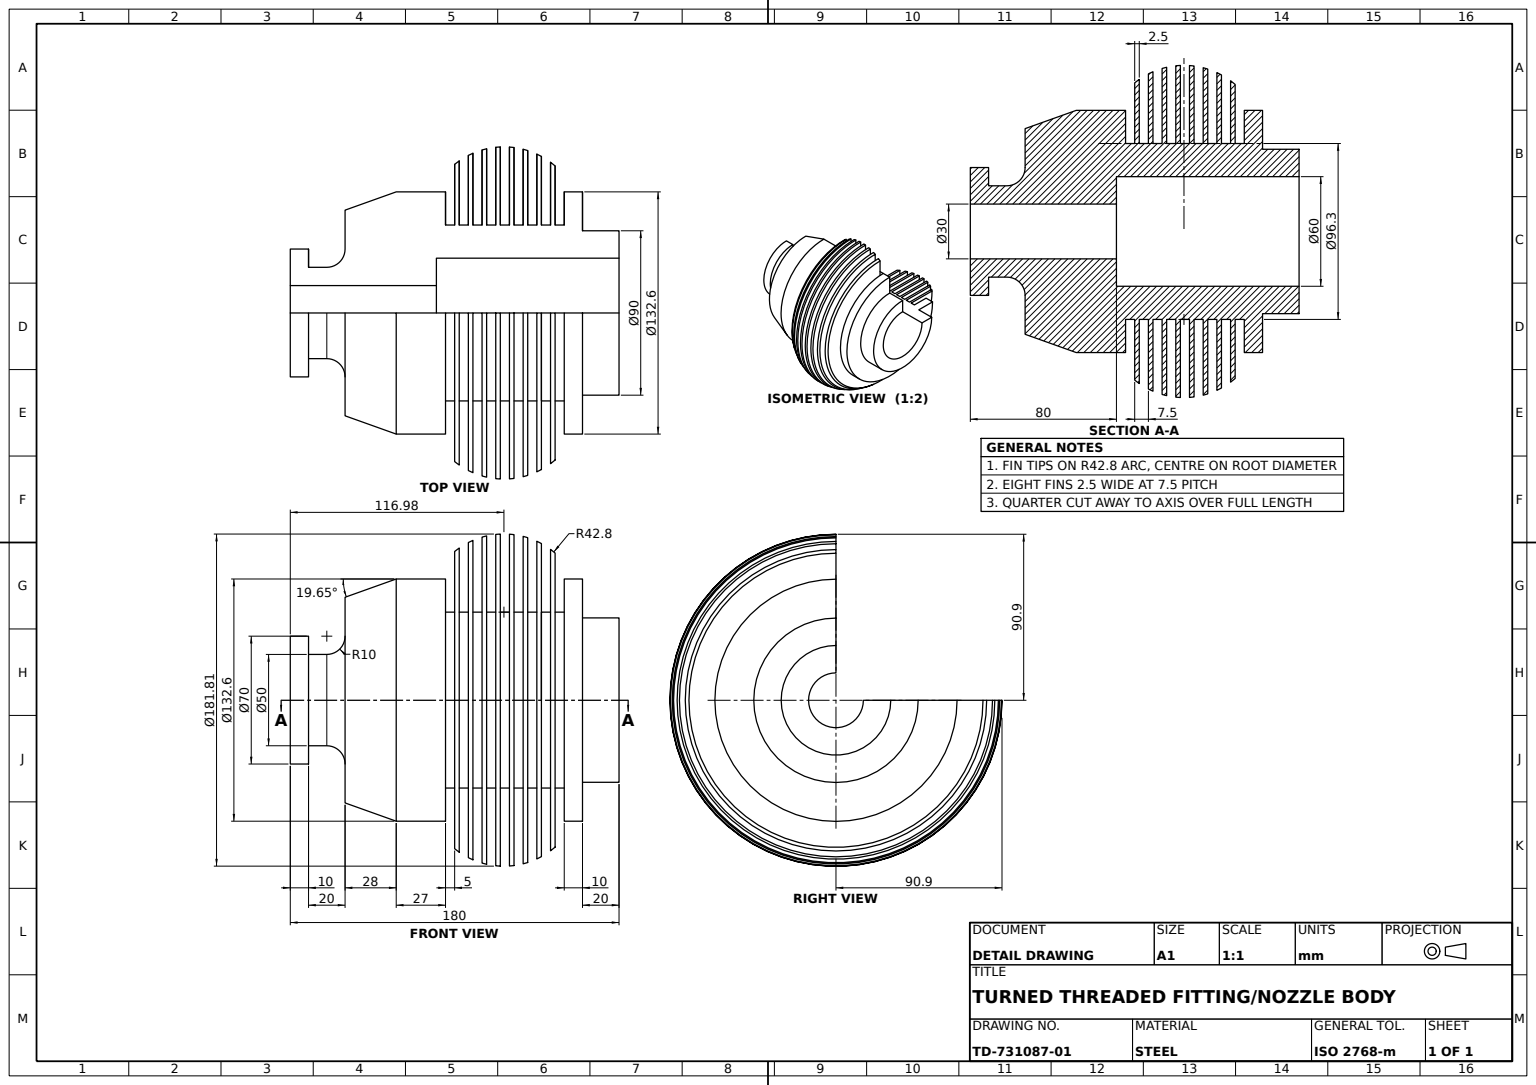
solid
v1 (31.156388,0,59.625514)
v2 (21.156388,0,59.625514)
e1 v1 v2 LINE
v3 (31.156388,66.3,-6.674486)
e2 v1 v3 CIRCLE(AX(P(31.156388,0,-6.674486),D(-1,0,0),D(0,0,1)),66.3)
v4 (21.156388,66.3,-6.674486)
e3 v3 v4 LINE
e4 v2 v4 CIRCLE(AX(P(21.156388,0,-6.674486),D(-1,0,0),D(0,0,1)),66.3)
face CYL(AX(P(-149.60578,0,-6.674486),D(-1,0,0),D(0,0,1)),66.3) [-e1 e2 e3 -e4]
v5 (-31.343612,0,41.475514)
v6 (-31.343612,48.15,-6.674486)
e5 v5 v6 CIRCLE(AX(P(-31.343612,0,-6.674486),D(-1,0,0),D(0,0,1)),48.15)
v7 (-36.343612,48.15,-6.674486)
e6 v7 v6 LINE
v8 (-36.343612,0,41.475514)
e7 v8 v7 CIRCLE(AX(P(-36.343612,0,-6.674486),D(-1,0,0),D(0,0,1)),48.15)
e8 v5 v8 LINE
face CYL(AX(P(-149.60578,0,-6.674486),D(-1,0,0),D(0,0,1)),48.15) [e5 -e6 -e7 -e8]
v9 (-13.843612,0,-54.824486)
v10 (-13.843612,0,41.475514)
e9 v9 v10 CIRCLE(AX(P(-13.843612,0,-6.674486),D(-1,0,0),D(0,0,1)),48.15)
v11 (-8.843612,0,-54.824486)
e10 v9 v11 LINE
v12 (-8.843612,0,41.475514)
e11 v11 v12 CIRCLE(AX(P(-8.843612,0,-6.674486),D(-1,0,0),D(0,0,1)),48.15)
e12 v12 v10 LINE
face CYL(AX(P(-149.60578,0,-6.674486),D(-1,0,0),D(0,0,1)),48.15) [-e9 e10 e11 e12]
v13 (-108.843612,0,18.325514)
v14 (-108.843612,25,-6.674486)
e13 v13 v14 CIRCLE(AX(P(-108.843612,0,-6.674486),D(-1,0,0),D(0,0,1)),25)
v15 (-98.843612,0,28.325514)
e14 v13 v15 CIRCLE(AX(P(-108.843612,0,28.325514),D(0,-1,0),D(0,0,-1)),10)
v16 (-98.843612,35,-6.674486)
e15 v15 v16 CIRCLE(AX(P(-98.843612,0,-6.674486),D(-1,0,0),D(0,0,1)),35)
e16 v16 v14 CIRCLE(AX(P(-108.843612,35,-6.674486),D(0,0,-1),D(1,0,0)),10)
face TORUS(AX(P(-108.843612,0,-6.674486),D(-1,0,0),D(0,0,1)),35,10) rev [-e13 e14 e15 e16]
v17 (6.156388,0,-54.824486)
v18 (6.156388,0,41.475514)
e17 v17 v18 CIRCLE(AX(P(6.156388,0,-6.674486),D(-1,0,0),D(0,0,1)),48.15)
v19 (1.156388,0,41.475514)
e18 v18 v19 LINE
v20 (1.156388,0,-54.824486)
e19 v20 v19 CIRCLE(AX(P(1.156388,0,-6.674486),D(-1,0,0),D(0,0,1)),48.15)
e20 v20 v17 LINE
face CYL(AX(P(-149.60578,0,-6.674486),D(-1,0,0),D(0,0,1)),48.15) [e17 e18 -e19 e20]
v21 (-128.843612,0,8.325514)
v22 (-128.843612,15,-6.674486)
e21 v21 v22 CIRCLE(AX(P(-128.843612,0,-6.674486),D(-1,0,0),D(0,0,1)),15)
v23 (-48.843612,15,-6.674486)
e22 v23 v22 LINE
v24 (-48.843612,0,8.325514)
e23 v24 v23 CIRCLE(AX(P(-48.843612,0,-6.674486),D(-1,0,0),D(0,0,1)),15)
e24 v24 v21 LINE
face CYL(AX(P(-149.60578,0,-6.674486),D(-1,0,0),D(0,0,1)),15) rev [e21 -e22 -e23 e24]
v25 (1.156388,0,-95.595676)
v26 (1.156388,0,82.246704)
e25 v25 v26 CIRCLE(AX(P(1.156388,0,-6.674486),D(-1,0,0),D(0,0,1)),88.92119)
e26 v25 v20 LINE
v27 (1.156388,48.15,-6.674486)
e27 v19 v27 CIRCLE(AX(P(1.156388,0,-6.674486),D(-1,0,0),D(0,0,1)),48.15)
v28 (1.156388,88.92119,-6.674486)
e28 v28 v27 LINE
e29 v26 v28 CIRCLE(AX(P(1.156388,0,-6.674486),D(-1,0,0),D(0,0,1)),88.92119)
face PLANE(AX(P(1.156388,0,0),D(1,0,0),D(0,0,-1))) [-e25 e26 e19 e27 -e28 -e29]
v29 (8.656388,0,79.035105)
v30 (8.656388,85.709591,-6.674486)
e30 v29 v30 CIRCLE(AX(P(8.656388,0,-6.674486),D(-1,0,0),D(0,0,1)),85.709591)
v31 (6.156388,86.97111,-6.674486)
e31 v30 v31 CIRCLE(AX(P(-11.86475,48.15,-6.674486),D(0,0,1),D(1,0,0)),42.8)
v32 (6.156388,0,80.296624)
e32 v32 v31 CIRCLE(AX(P(6.156388,0,-6.674486),D(-1,0,0),D(0,0,1)),86.97111)
e33 v29 v32 CIRCLE(AX(P(-11.86475,0,41.475514),D(0,-1,0),D(0,0,-1)),42.8)
face TORUS(AX(P(-11.86475,0,-6.674486),D(-1,0,0),D(0,0,1)),48.15,42.8) [e30 e31 -e32 -e33]
v33 (-6.343612,0,-54.824486)
v34 (-1.343612,0,-54.824486)
e34 v33 v34 LINE
v35 (-1.343612,0,41.475514)
e35 v34 v35 CIRCLE(AX(P(-1.343612,0,-6.674486),D(-1,0,0),D(0,0,1)),48.15)
v36 (-6.343612,0,41.475514)
e36 v35 v36 LINE
e37 v33 v36 CIRCLE(AX(P(-6.343612,0,-6.674486),D(-1,0,0),D(0,0,1)),48.15)
face CYL(AX(P(-149.60578,0,-6.674486),D(-1,0,0),D(0,0,1)),48.15) [e34 e35 e36 -e37]
v37 (-108.843612,0,-31.674486)
e38 v37 v13 CIRCLE(AX(P(-108.843612,0,-6.674486),D(-1,0,0),D(0,0,1)),25)
v38 (-98.843612,0,-41.674486)
e39 v38 v37 CIRCLE(AX(P(-108.843612,0,-41.674486),D(0,-1,0),D(0,0,1)),10)
e40 v38 v15 CIRCLE(AX(P(-98.843612,0,-6.674486),D(-1,0,0),D(0,0,1)),35)
face TORUS(AX(P(-108.843612,0,-6.674486),D(-1,0,0),D(0,0,1)),35,10) rev [-e38 -e39 e40 -e14]
v39 (-128.843612,0,-41.674486)
v40 (-128.843612,0,28.325514)
e41 v39 v40 CIRCLE(AX(P(-128.843612,0,-6.674486),D(-1,0,0),D(0,0,1)),35)
v41 (-118.843612,0,-41.674486)
e42 v39 v41 LINE
v42 (-118.843612,0,28.325514)
e43 v41 v42 CIRCLE(AX(P(-118.843612,0,-6.674486),D(-1,0,0),D(0,0,1)),35)
e44 v42 v40 LINE
face CYL(AX(P(-149.60578,0,-6.674486),D(-1,0,0),D(0,0,1)),35) [-e41 e42 e43 e44]
v43 (-13.843612,48.15,-6.674486)
e45 v10 v43 CIRCLE(AX(P(-13.843612,0,-6.674486),D(-1,0,0),D(0,0,1)),48.15)
v44 (-8.843612,48.15,-6.674486)
e46 v12 v44 CIRCLE(AX(P(-8.843612,0,-6.674486),D(-1,0,0),D(0,0,1)),48.15)
e47 v43 v44 LINE
face CYL(AX(P(-149.60578,0,-6.674486),D(-1,0,0),D(0,0,1)),48.15) [-e45 -e12 e46 -e47]
v45 (-43.843612,0,-72.974486)
v46 (-70.843612,0,-72.974486)
e48 v45 v46 LINE
v47 (-43.843612,0,59.625514)
e49 v45 v47 CIRCLE(AX(P(-43.843612,0,-6.674486),D(-1,0,0),D(0,0,1)),66.3)
v48 (-70.843612,0,59.625514)
e50 v47 v48 LINE
e51 v46 v48 CIRCLE(AX(P(-70.843612,0,-6.674486),D(-1,0,0),D(0,0,1)),66.3)
face CYL(AX(P(-149.60578,0,-6.674486),D(-1,0,0),D(0,0,1)),66.3) [-e48 e49 e50 -e51]
v49 (-128.843612,0,-21.674486)
e52 v49 v21 CIRCLE(AX(P(-128.843612,0,-6.674486),D(-1,0,0),D(0,0,1)),15)
v50 (-48.843612,0,-21.674486)
e53 v50 v24 CIRCLE(AX(P(-48.843612,0,-6.674486),D(-1,0,0),D(0,0,1)),15)
e54 v50 v49 LINE
face CYL(AX(P(-149.60578,0,-6.674486),D(-1,0,0),D(0,0,1)),15) rev [e52 -e24 -e53 e54]
v51 (-1.343612,0,82.962207)
e55 v26 v51 CIRCLE(AX(P(-11.86475,0,41.475514),D(0,-1,0),D(0,0,-1)),42.8)
v52 (-1.343612,0,-96.311178)
e56 v52 v51 CIRCLE(AX(P(-1.343612,0,-6.674486),D(-1,0,0),D(0,0,1)),89.636692)
e57 v25 v52 CIRCLE(AX(P(-11.86475,0,-54.824486),D(0,1,0),D(0,0,1)),42.8)
face TORUS(AX(P(-11.86475,0,-6.674486),D(-1,0,0),D(0,0,1)),48.15,42.8) [e55 -e56 -e57 e25]
v53 (-13.843612,90.904229,-6.674486)
e58 v43 v53 LINE
v54 (-13.843612,0,84.229743)
e59 v54 v53 CIRCLE(AX(P(-13.843612,0,-6.674486),D(-1,0,0),D(0,0,1)),90.904229)
v55 (-13.843612,0,-97.578715)
e60 v55 v54 CIRCLE(AX(P(-13.843612,0,-6.674486),D(-1,0,0),D(0,0,1)),90.904229)
e61 v9 v55 LINE
face PLANE(AX(P(-13.843612,0,-75.255525),D(-1,0,0),D(0,0,1))) rev [e9 e45 e58 -e59 -e60 -e61]
v56 (-48.843612,0,23.325514)
v57 (-48.843612,30,-6.674486)
e62 v56 v57 CIRCLE(AX(P(-48.843612,0,-6.674486),D(-1,0,0),D(0,0,1)),30)
v58 (51.156388,30,-6.674486)
e63 v58 v57 LINE
v59 (51.156388,0,23.325514)
e64 v59 v58 CIRCLE(AX(P(51.156388,0,-6.674486),D(-1,0,0),D(0,0,1)),30)
e65 v59 v56 LINE
face CYL(AX(P(-149.60578,0,-6.674486),D(-1,0,0),D(0,0,1)),30) rev [e62 -e63 -e64 e65]
v60 (-21.343612,0,-54.824486)
v61 (-21.343612,0,41.475514)
e66 v60 v61 CIRCLE(AX(P(-21.343612,0,-6.674486),D(-1,0,0),D(0,0,1)),48.15)
v62 (-21.343612,48.15,-6.674486)
e67 v61 v62 CIRCLE(AX(P(-21.343612,0,-6.674486),D(-1,0,0),D(0,0,1)),48.15)
v63 (-21.343612,89.887168,-6.674486)
e68 v62 v63 LINE
v64 (-21.343612,0,83.212682)
e69 v64 v63 CIRCLE(AX(P(-21.343612,0,-6.674486),D(-1,0,0),D(0,0,1)),89.887168)
v65 (-21.343612,0,-96.561654)
e70 v65 v64 CIRCLE(AX(P(-21.343612,0,-6.674486),D(-1,0,0),D(0,0,1)),89.887168)
e71 v60 v65 LINE
face PLANE(AX(P(-21.343612,0,0),D(-1,0,0),D(0,0,1))) rev [e66 e67 e68 -e69 -e70 -e71]
v66 (16.156388,0,-87.176546)
v67 (13.656388,0,-89.183058)
e72 v66 v67 CIRCLE(AX(P(-11.86475,0,-54.824486),D(0,1,0),D(0,0,1)),42.8)
v68 (16.156388,0,73.827574)
e73 v66 v68 CIRCLE(AX(P(16.156388,0,-6.674486),D(-1,0,0),D(0,0,1)),80.50206)
v69 (13.656388,0,75.834087)
e74 v68 v69 CIRCLE(AX(P(-11.86475,0,41.475514),D(0,-1,0),D(0,0,-1)),42.8)
e75 v67 v69 CIRCLE(AX(P(13.656388,0,-6.674486),D(-1,0,0),D(0,0,1)),82.508572)
face TORUS(AX(P(-11.86475,0,-6.674486),D(-1,0,0),D(0,0,1)),48.15,42.8) [-e72 e73 e74 -e75]
v70 (-118.843612,0,-31.674486)
v71 (-118.843612,0,18.325514)
e76 v70 v71 CIRCLE(AX(P(-118.843612,0,-6.674486),D(-1,0,0),D(0,0,1)),25)
v72 (-118.843612,25,-6.674486)
e77 v71 v72 CIRCLE(AX(P(-118.843612,0,-6.674486),D(-1,0,0),D(0,0,1)),25)
v73 (-118.843612,35,-6.674486)
e78 v73 v72 LINE
e79 v42 v73 CIRCLE(AX(P(-118.843612,0,-6.674486),D(-1,0,0),D(0,0,1)),35)
e80 v41 v70 LINE
face PLANE(AX(P(-118.843612,0,0),D(1,0,0),D(0,0,-1))) [e76 e77 -e78 -e79 -e43 e80]
v74 (-28.843612,0,-94.11263)
v75 (-31.343612,0,-92.935035)
e81 v74 v75 CIRCLE(AX(P(-11.86475,0,-54.824486),D(0,1,0),D(0,0,1)),42.8)
v76 (-28.843612,0,80.763658)
e82 v74 v76 CIRCLE(AX(P(-28.843612,0,-6.674486),D(-1,0,0),D(0,0,1)),87.438144)
v77 (-31.343612,0,79.586063)
e83 v76 v77 CIRCLE(AX(P(-11.86475,0,41.475514),D(0,-1,0),D(0,0,-1)),42.8)
e84 v75 v77 CIRCLE(AX(P(-31.343612,0,-6.674486),D(-1,0,0),D(0,0,1)),86.260549)
face TORUS(AX(P(-11.86475,0,-6.674486),D(-1,0,0),D(0,0,1)),48.15,42.8) [-e81 e82 e83 -e84]
v78 (-16.343612,0,41.475514)
e85 v78 v61 LINE
v79 (-16.343612,0,-54.824486)
e86 v60 v79 LINE
e87 v79 v78 CIRCLE(AX(P(-16.343612,0,-6.674486),D(-1,0,0),D(0,0,1)),48.15)
face CYL(AX(P(-149.60578,0,-6.674486),D(-1,0,0),D(0,0,1)),48.15) [e85 -e66 e86 e87]
e88 v72 v14 LINE
e89 v13 v71 LINE
face CYL(AX(P(-149.60578,0,-6.674486),D(-1,0,0),D(0,0,1)),25) [e13 -e88 -e77 -e89]
v80 (16.156388,0,-54.824486)
e90 v80 v66 LINE
v81 (16.156388,0,41.475514)
e91 v80 v81 CIRCLE(AX(P(16.156388,0,-6.674486),D(-1,0,0),D(0,0,1)),48.15)
v82 (16.156388,48.15,-6.674486)
e92 v81 v82 CIRCLE(AX(P(16.156388,0,-6.674486),D(-1,0,0),D(0,0,1)),48.15)
v83 (16.156388,80.50206,-6.674486)
e93 v82 v83 LINE
e94 v68 v83 CIRCLE(AX(P(16.156388,0,-6.674486),D(-1,0,0),D(0,0,1)),80.50206)
face PLANE(AX(P(16.156388,0,0),D(-1,0,0),D(0,0,1))) rev [-e73 -e90 e91 e92 e93 -e94]
v84 (-28.843612,0,41.475514)
v85 (-28.843612,48.15,-6.674486)
e95 v84 v85 CIRCLE(AX(P(-28.843612,0,-6.674486),D(-1,0,0),D(0,0,1)),48.15)
v86 (-23.843612,0,41.475514)
e96 v86 v84 LINE
v87 (-23.843612,48.15,-6.674486)
e97 v86 v87 CIRCLE(AX(P(-23.843612,0,-6.674486),D(-1,0,0),D(0,0,1)),48.15)
e98 v85 v87 LINE
face CYL(AX(P(-149.60578,0,-6.674486),D(-1,0,0),D(0,0,1)),48.15) [-e95 -e96 e97 -e98]
v88 (-128.843612,35,-6.674486)
e99 v40 v88 CIRCLE(AX(P(-128.843612,0,-6.674486),D(-1,0,0),D(0,0,1)),35)
e100 v22 v88 LINE
e101 v49 v39 LINE
face PLANE(AX(P(-128.843612,0,0),D(-1,0,0),D(0,0,1))) [e41 e99 -e100 -e21 -e52 e101]
v89 (8.656388,0,-92.384077)
v90 (6.156388,0,-93.645596)
e102 v89 v90 CIRCLE(AX(P(-11.86475,0,-54.824486),D(0,1,0),D(0,0,1)),42.8)
e103 v89 v29 CIRCLE(AX(P(8.656388,0,-6.674486),D(-1,0,0),D(0,0,1)),85.709591)
e104 v90 v32 CIRCLE(AX(P(6.156388,0,-6.674486),D(-1,0,0),D(0,0,1)),86.97111)
face TORUS(AX(P(-11.86475,0,-6.674486),D(-1,0,0),D(0,0,1)),48.15,42.8) [-e102 e103 e33 -e104]
v91 (-6.343612,48.15,-6.674486)
v92 (-6.343612,90.592397,-6.674486)
e105 v91 v92 LINE
v93 (-6.343612,0,83.917911)
e106 v93 v92 CIRCLE(AX(P(-6.343612,0,-6.674486),D(-1,0,0),D(0,0,1)),90.592397)
v94 (-6.343612,0,-97.266882)
e107 v94 v93 CIRCLE(AX(P(-6.343612,0,-6.674486),D(-1,0,0),D(0,0,1)),90.592397)
e108 v33 v94 LINE
e109 v36 v91 CIRCLE(AX(P(-6.343612,0,-6.674486),D(-1,0,0),D(0,0,1)),48.15)
face PLANE(AX(P(-6.343612,0,-75.255525),D(-1,0,0),D(0,0,1))) rev [e105 -e106 -e107 -e108 e37 e109]
e110 v57 v23 LINE
e111 v88 v73 LINE
v95 (-98.843612,56.3,-6.674486)
e112 v16 v95 LINE
v96 (-70.843612,66.3,-6.674486)
e113 v96 v95 LINE
v97 (-43.843612,66.3,-6.674486)
e114 v97 v96 LINE
v98 (-43.843612,48.15,-6.674486)
e115 v97 v98 LINE
v99 (-38.843612,48.15,-6.674486)
e116 v98 v99 LINE
v100 (-38.843612,81.37621,-6.674486)
e117 v99 v100 LINE
v101 (-36.343612,83.258764,-6.674486)
e118 v101 v100 CIRCLE(AX(P(-11.86475,48.15,-6.674486),D(0,0,1),D(1,0,0)),42.8)
e119 v101 v7 LINE
v102 (-31.343612,86.260549,-6.674486)
e120 v6 v102 LINE
v103 (-28.843612,87.438144,-6.674486)
e121 v103 v102 CIRCLE(AX(P(-11.86475,48.15,-6.674486),D(0,0,1),D(1,0,0)),42.8)
e122 v103 v85 LINE
v104 (-23.843612,89.239498,-6.674486)
e123 v87 v104 LINE
e124 v63 v104 CIRCLE(AX(P(-11.86475,48.15,-6.674486),D(0,0,1),D(1,0,0)),42.8)
v105 (-16.343612,48.15,-6.674486)
e125 v62 v105 LINE
v106 (-16.343612,90.715007,-6.674486)
e126 v106 v105 LINE
e127 v53 v106 CIRCLE(AX(P(-11.86475,48.15,-6.674486),D(0,0,1),D(1,0,0)),42.8)
v107 (-8.843612,90.84324,-6.674486)
e128 v107 v44 LINE
e129 v92 v107 CIRCLE(AX(P(-11.86475,48.15,-6.674486),D(0,0,1),D(1,0,0)),42.8)
v108 (-1.343612,48.15,-6.674486)
e130 v91 v108 LINE
v109 (-1.343612,89.636692,-6.674486)
e131 v108 v109 LINE
e132 v28 v109 CIRCLE(AX(P(-11.86475,48.15,-6.674486),D(0,0,1),D(1,0,0)),42.8)
v110 (6.156388,48.15,-6.674486)
e133 v27 v110 LINE
e134 v110 v31 LINE
v111 (8.656388,48.15,-6.674486)
e135 v30 v111 LINE
v112 (13.656388,48.15,-6.674486)
e136 v111 v112 LINE
v113 (13.656388,82.508572,-6.674486)
e137 v112 v113 LINE
e138 v83 v113 CIRCLE(AX(P(-11.86475,48.15,-6.674486),D(0,0,1),D(1,0,0)),42.8)
v114 (21.156388,48.15,-6.674486)
e139 v82 v114 LINE
e140 v4 v114 LINE
v115 (31.156388,45,-6.674486)
e141 v115 v3 LINE
v116 (51.156388,45,-6.674486)
e142 v116 v115 LINE
e143 v58 v116 LINE
face PLANE(AX(P(132.156388,0,-6.674486),D(0,0,1),D(1,0,0))) rev [e63 e110 e22 e100 e111 e78 e88 -e16 e112 -e113 -e114 e115 e116 e117 -e118 e119 e6 e120 -e121 e122 e98 e123 -e124 -e68 e125 -e126 -e127 -e58 e47 -e128 -e129 -e105 e130 e131 -e132 e28 e133 e134 -e31 e135 e136 e137 -e138 -e93 e139 -e140 -e3 -e141 -e142 -e143]
v117 (-23.843612,0,-95.913984)
e144 v65 v117 CIRCLE(AX(P(-11.86475,0,-54.824486),D(0,1,0),D(0,0,1)),42.8)
v118 (-23.843612,0,82.565013)
e145 v64 v118 CIRCLE(AX(P(-11.86475,0,41.475514),D(0,-1,0),D(0,0,-1)),42.8)
e146 v117 v118 CIRCLE(AX(P(-23.843612,0,-6.674486),D(-1,0,0),D(0,0,1)),89.239498)
face TORUS(AX(P(-11.86475,0,-6.674486),D(-1,0,0),D(0,0,1)),48.15,42.8) [-e144 e70 e145 -e146]
v119 (-38.843612,0,41.475514)
e147 v119 v99 CIRCLE(AX(P(-38.843612,0,-6.674486),D(-1,0,0),D(0,0,1)),48.15)
v120 (-38.843612,0,-54.824486)
e148 v120 v119 CIRCLE(AX(P(-38.843612,0,-6.674486),D(-1,0,0),D(0,0,1)),48.15)
v121 (-38.843612,0,-88.050696)
e149 v120 v121 LINE
v122 (-38.843612,0,74.701724)
e150 v121 v122 CIRCLE(AX(P(-38.843612,0,-6.674486),D(-1,0,0),D(0,0,1)),81.37621)
e151 v122 v100 CIRCLE(AX(P(-38.843612,0,-6.674486),D(-1,0,0),D(0,0,1)),81.37621)
face PLANE(AX(P(-38.843612,0,0),D(-1,0,0),D(0,0,1))) [-e117 -e147 -e148 e149 e150 e151]
v123 (31.156388,0,-51.674486)
v124 (31.156388,0,38.325514)
e152 v123 v124 CIRCLE(AX(P(31.156388,0,-6.674486),D(-1,0,0),D(0,0,1)),45)
e153 v124 v115 CIRCLE(AX(P(31.156388,0,-6.674486),D(-1,0,0),D(0,0,1)),45)
v125 (31.156388,0,-72.974486)
e154 v125 v1 CIRCLE(AX(P(31.156388,0,-6.674486),D(-1,0,0),D(0,0,1)),66.3)
e155 v123 v125 LINE
face PLANE(AX(P(31.156388,0,0),D(-1,0,0),D(0,0,1))) rev [e152 e153 e141 -e2 -e154 -e155]
v126 (-23.843612,0,-54.824486)
e156 v126 v86 CIRCLE(AX(P(-23.843612,0,-6.674486),D(-1,0,0),D(0,0,1)),48.15)
v127 (-28.843612,0,-54.824486)
e157 v127 v84 CIRCLE(AX(P(-28.843612,0,-6.674486),D(-1,0,0),D(0,0,1)),48.15)
e158 v127 v126 LINE
face CYL(AX(P(-149.60578,0,-6.674486),D(-1,0,0),D(0,0,1)),48.15) [e156 e96 -e157 e158]
v128 (-43.843612,0,-54.824486)
v129 (-43.843612,0,41.475514)
e159 v128 v129 CIRCLE(AX(P(-43.843612,0,-6.674486),D(-1,0,0),D(0,0,1)),48.15)
e160 v129 v98 CIRCLE(AX(P(-43.843612,0,-6.674486),D(-1,0,0),D(0,0,1)),48.15)
e161 v47 v97 CIRCLE(AX(P(-43.843612,0,-6.674486),D(-1,0,0),D(0,0,1)),66.3)
e162 v45 v128 LINE
face PLANE(AX(P(-43.843612,0,0),D(1,0,0),D(0,0,-1))) [e159 e160 -e115 -e161 -e49 e162]
e163 v76 v103 CIRCLE(AX(P(-28.843612,0,-6.674486),D(-1,0,0),D(0,0,1)),87.438144)
e164 v74 v127 LINE
face PLANE(AX(P(-28.843612,0,0),D(1,0,0),D(0,0,-1))) [-e163 -e82 e164 e157 e95 -e122]
e165 v119 v129 LINE
e166 v128 v120 LINE
face CYL(AX(P(-149.60578,0,-6.674486),D(-1,0,0),D(0,0,1)),48.15) [e165 -e159 e166 e148]
v130 (-36.343612,0,-54.824486)
e167 v130 v8 CIRCLE(AX(P(-36.343612,0,-6.674486),D(-1,0,0),D(0,0,1)),48.15)
v131 (-36.343612,0,76.584279)
e168 v131 v101 CIRCLE(AX(P(-36.343612,0,-6.674486),D(-1,0,0),D(0,0,1)),83.258764)
v132 (-36.343612,0,-89.93325)
e169 v132 v131 CIRCLE(AX(P(-36.343612,0,-6.674486),D(-1,0,0),D(0,0,1)),83.258764)
e170 v132 v130 LINE
face PLANE(AX(P(-36.343612,0,0),D(1,0,0),D(0,0,-1))) [e167 e7 -e119 -e168 -e169 e170]
v133 (-31.343612,0,-54.824486)
e171 v130 v133 LINE
e172 v133 v5 CIRCLE(AX(P(-31.343612,0,-6.674486),D(-1,0,0),D(0,0,1)),48.15)
face CYL(AX(P(-149.60578,0,-6.674486),D(-1,0,0),D(0,0,1)),48.15) [e8 -e167 e171 e172]
v134 (-16.343612,0,-97.389493)
e173 v134 v79 LINE
v135 (-16.343612,0,84.040521)
e174 v134 v135 CIRCLE(AX(P(-16.343612,0,-6.674486),D(-1,0,0),D(0,0,1)),90.715007)
e175 v135 v106 CIRCLE(AX(P(-16.343612,0,-6.674486),D(-1,0,0),D(0,0,1)),90.715007)
e176 v78 v105 CIRCLE(AX(P(-16.343612,0,-6.674486),D(-1,0,0),D(0,0,1)),48.15)
face PLANE(AX(P(-16.343612,0,-75.255525),D(1,0,0),D(0,0,-1))) rev [-e87 -e173 e174 e175 e126 -e176]
v136 (13.656388,0,41.475514)
e177 v136 v112 CIRCLE(AX(P(13.656388,0,-6.674486),D(-1,0,0),D(0,0,1)),48.15)
v137 (13.656388,0,-54.824486)
e178 v137 v136 CIRCLE(AX(P(13.656388,0,-6.674486),D(-1,0,0),D(0,0,1)),48.15)
e179 v137 v67 LINE
e180 v69 v113 CIRCLE(AX(P(13.656388,0,-6.674486),D(-1,0,0),D(0,0,1)),82.508572)
face PLANE(AX(P(13.656388,0,0),D(-1,0,0),D(0,0,1))) [-e177 -e178 e179 e75 e180 -e137]
face CYL(AX(P(-149.60578,0,-6.674486),D(-1,0,0),D(0,0,1)),48.15) [e147 -e116 -e160 -e165]
e181 v51 v109 CIRCLE(AX(P(-1.343612,0,-6.674486),D(-1,0,0),D(0,0,1)),89.636692)
face TORUS(AX(P(-11.86475,0,-6.674486),D(-1,0,0),D(0,0,1)),48.15,42.8) [e132 -e181 -e55 e29]
v138 (51.156388,0,-36.674486)
e182 v138 v59 CIRCLE(AX(P(51.156388,0,-6.674486),D(-1,0,0),D(0,0,1)),30)
v139 (-48.843612,0,-36.674486)
e183 v138 v139 LINE
e184 v139 v56 CIRCLE(AX(P(-48.843612,0,-6.674486),D(-1,0,0),D(0,0,1)),30)
face CYL(AX(P(-149.60578,0,-6.674486),D(-1,0,0),D(0,0,1)),30) rev [-e182 e183 e184 -e65]
v140 (51.156388,0,-51.674486)
e185 v140 v123 LINE
v141 (51.156388,0,38.325514)
e186 v140 v141 CIRCLE(AX(P(51.156388,0,-6.674486),D(-1,0,0),D(0,0,1)),45)
e187 v141 v124 LINE
face CYL(AX(P(-149.60578,0,-6.674486),D(-1,0,0),D(0,0,1)),45) [-e185 e186 e187 -e152]
e188 v70 v37 LINE
face CYL(AX(P(-149.60578,0,-6.674486),D(-1,0,0),D(0,0,1)),25) [-e76 e188 e38 e89]
e189 v34 v52 LINE
e190 v35 v108 CIRCLE(AX(P(-1.343612,0,-6.674486),D(-1,0,0),D(0,0,1)),48.15)
face PLANE(AX(P(-1.343612,0,0),D(-1,0,0),D(0,0,1))) [-e35 e189 e56 e181 -e131 -e190]
v142 (-8.843612,0,-97.517726)
v143 (-8.843612,0,84.168754)
e191 v142 v143 CIRCLE(AX(P(-8.843612,0,-6.674486),D(-1,0,0),D(0,0,1)),90.84324)
e192 v94 v142 CIRCLE(AX(P(-11.86475,0,-54.824486),D(0,1,0),D(0,0,1)),42.8)
e193 v93 v143 CIRCLE(AX(P(-11.86475,0,41.475514),D(0,-1,0),D(0,0,-1)),42.8)
face TORUS(AX(P(-11.86475,0,-6.674486),D(-1,0,0),D(0,0,1)),48.15,42.8) [-e191 -e192 e107 e193]
face CYL(AX(P(-149.60578,0,-6.674486),D(-1,0,0),D(0,0,1)),35) [-e111 -e99 -e44 e79]
e194 v54 v135 CIRCLE(AX(P(-11.86475,0,41.475514),D(0,-1,0),D(0,0,-1)),42.8)
e195 v55 v134 CIRCLE(AX(P(-11.86475,0,-54.824486),D(0,1,0),D(0,0,1)),42.8)
face TORUS(AX(P(-11.86475,0,-6.674486),D(-1,0,0),D(0,0,1)),48.15,42.8) [e60 e194 -e174 -e195]
e196 v138 v140 LINE
e197 v141 v116 CIRCLE(AX(P(51.156388,0,-6.674486),D(-1,0,0),D(0,0,1)),45)
face PLANE(AX(P(51.156388,0,0),D(-1,0,0),D(0,0,1))) rev [-e186 -e196 e182 e64 e143 -e197]
v144 (-98.843612,0,-62.974486)
e198 v38 v144 LINE
e199 v144 v95 CIRCLE(AX(P(-98.843612,0,-6.674486),D(-1,0,0),D(0,0,1)),56.3)
face PLANE(AX(P(-98.843612,0,0),D(-1,0,0),D(0,0,1))) [e198 e199 -e112 -e15 -e40]
v145 (21.156388,0,-72.974486)
e200 v125 v145 LINE
v146 (21.156388,0,-54.824486)
e201 v145 v146 LINE
e202 v80 v146 LINE
v147 (8.656388,0,-54.824486)
e203 v147 v137 LINE
e204 v89 v147 LINE
e205 v17 v90 LINE
e206 v142 v11 LINE
e207 v126 v117 LINE
e208 v133 v75 LINE
e209 v132 v121 CIRCLE(AX(P(-11.86475,0,-54.824486),D(0,1,0),D(0,0,1)),42.8)
e210 v46 v144 LINE
e211 v139 v50 LINE
face PLANE(AX(P(132.156388,0,0),D(0,1,0),D(0,0,1))) [e155 e200 e201 -e202 e90 e72 -e179 -e203 -e204 e102 -e205 -e20 -e26 e57 -e189 -e34 e108 e192 e206 -e10 e61 e195 e173 -e86 e71 e144 -e207 -e158 -e164 e81 -e208 -e171 -e170 e209 -e149 -e166 -e162 e48 e210 -e198 e39 -e188 -e80 -e42 -e101 -e54 -e211 -e183 e196 e185]
e212 v145 v2 CIRCLE(AX(P(21.156388,0,-6.674486),D(-1,0,0),D(0,0,1)),66.3)
face CYL(AX(P(-149.60578,0,-6.674486),D(-1,0,0),D(0,0,1)),66.3) [-e212 -e200 e154 e1]
e213 v77 v102 CIRCLE(AX(P(-31.343612,0,-6.674486),D(-1,0,0),D(0,0,1)),86.260549)
face PLANE(AX(P(-31.343612,0,0),D(-1,0,0),D(0,0,1))) [e84 e213 -e120 -e5 -e172 e208]
e214 v131 v122 CIRCLE(AX(P(-11.86475,0,41.475514),D(0,-1,0),D(0,0,-1)),42.8)
face TORUS(AX(P(-11.86475,0,-6.674486),D(-1,0,0),D(0,0,1)),48.15,42.8) [-e151 -e214 e168 e118]
e215 v143 v107 CIRCLE(AX(P(-8.843612,0,-6.674486),D(-1,0,0),D(0,0,1)),90.84324)
face TORUS(AX(P(-11.86475,0,-6.674486),D(-1,0,0),D(0,0,1)),48.15,42.8) [e106 e129 -e215 -e193]
v148 (21.156388,0,41.475514)
e216 v148 v81 LINE
e217 v148 v114 CIRCLE(AX(P(21.156388,0,-6.674486),D(-1,0,0),D(0,0,1)),48.15)
face CYL(AX(P(-149.60578,0,-6.674486),D(-1,0,0),D(0,0,1)),48.15) [-e92 -e216 e217 -e139]
e218 v18 v110 CIRCLE(AX(P(6.156388,0,-6.674486),D(-1,0,0),D(0,0,1)),48.15)
face CYL(AX(P(-149.60578,0,-6.674486),D(-1,0,0),D(0,0,1)),48.15) [-e18 e218 -e133 -e27]
v149 (8.656388,0,41.475514)
e219 v136 v149 LINE
e220 v147 v149 CIRCLE(AX(P(8.656388,0,-6.674486),D(-1,0,0),D(0,0,1)),48.15)
face CYL(AX(P(-149.60578,0,-6.674486),D(-1,0,0),D(0,0,1)),48.15) [e203 e178 e219 -e220]
e221 v118 v104 CIRCLE(AX(P(-23.843612,0,-6.674486),D(-1,0,0),D(0,0,1)),89.239498)
face TORUS(AX(P(-11.86475,0,-6.674486),D(-1,0,0),D(0,0,1)),48.15,42.8) [-e221 -e145 e69 e124]
face TORUS(AX(P(-11.86475,0,-6.674486),D(-1,0,0),D(0,0,1)),48.15,42.8) [e214 -e150 -e209 e169]
e222 v48 v96 CIRCLE(AX(P(-70.843612,0,-6.674486),D(-1,0,0),D(0,0,1)),66.3)
face CYL(AX(P(-149.60578,0,-6.674486),D(-1,0,0),D(0,0,1)),66.3) [-e50 e161 e114 -e222]
e223 v149 v111 CIRCLE(AX(P(8.656388,0,-6.674486),D(-1,0,0),D(0,0,1)),48.15)
face CYL(AX(P(-149.60578,0,-6.674486),D(-1,0,0),D(0,0,1)),48.15) [e177 -e136 -e223 -e219]
face CONE(AX(P(-70.843612,0,-6.674486),D(1,0,0),D(0,0,-1)),66.3,0.34302394) [-e199 -e210 e51 e222 e113]
face TORUS(AX(P(-11.86475,0,-6.674486),D(-1,0,0),D(0,0,1)),48.15,42.8) [-e180 -e74 e94 e138]
face PLANE(AX(P(-8.843612,0,-75.255525),D(1,0,0),D(0,0,-1))) rev [e191 e215 e128 -e46 -e11 -e206]
e224 v146 v148 CIRCLE(AX(P(21.156388,0,-6.674486),D(-1,0,0),D(0,0,1)),48.15)
face CYL(AX(P(-149.60578,0,-6.674486),D(-1,0,0),D(0,0,1)),48.15) [e224 e216 -e91 e202]
face PLANE(AX(P(6.156388,0,0),D(-1,0,0),D(0,0,1))) [-e218 -e17 e205 e104 e32 -e134]
face PLANE(AX(P(21.156388,0,0),D(1,0,0),D(0,0,-1))) rev [e212 e4 e140 -e217 -e224 -e201]
face CYL(AX(P(-149.60578,0,-6.674486),D(-1,0,0),D(0,0,1)),48.15) [-e109 -e36 e190 -e130]
face TORUS(AX(P(-11.86475,0,-6.674486),D(-1,0,0),D(0,0,1)),48.15,42.8) [-e175 -e194 e59 e127]
face PLANE(AX(P(-23.843612,0,0),D(-1,0,0),D(0,0,1))) [e221 -e123 -e97 -e156 e207 e146]
face TORUS(AX(P(-11.86475,0,-6.674486),D(-1,0,0),D(0,0,1)),48.15,42.8) [-e83 e163 e121 -e213]
face CYL(AX(P(-149.60578,0,-6.674486),D(-1,0,0),D(0,0,1)),48.15) [-e85 e176 -e125 -e67]
face PLANE(AX(P(8.656388,0,0),D(1,0,0),D(0,0,-1))) [e223 -e135 -e30 -e103 e204 e220]
face CYL(AX(P(-149.60578,0,-6.674486),D(-1,0,0),D(0,0,1)),45) [e197 e142 -e153 -e187]
face PLANE(AX(P(-48.843612,0,0),D(1,0,0),D(0,0,-1))) [-e110 -e62 -e184 e211 e53 e23]
